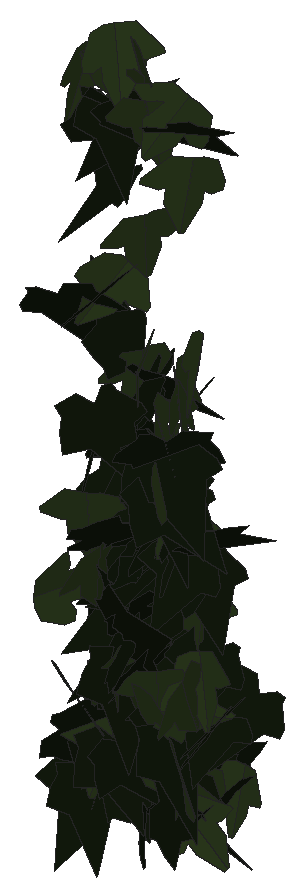
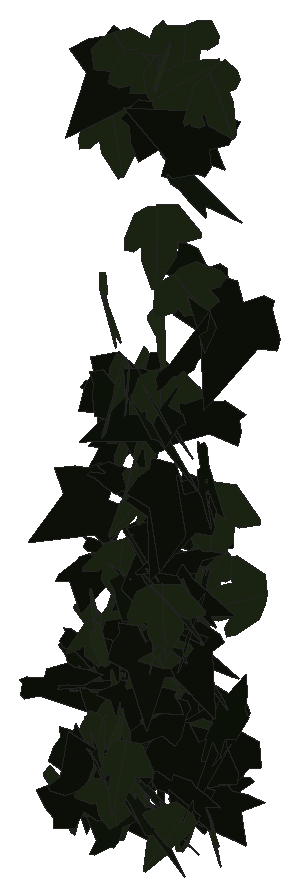
# SketchUp Ruby script. Lengths in inches.
U = 1.inch
M = Sketchup.active_model
def pt(a) = Geom::Point3d.new(a.map { |v| v * U })
def face(e, loops, mat)
  f = e.add_face(loops[0].map { |a| pt(a) })
  loops[1..].each { |l| e.add_face(l.map { |a| pt(a) }).erase! }
  f.material = f.back_material = mat if mat
  f
end
# faces: each face lists its corners as indices into pts; further lists are holes
def faces(e, pts, list, mat = nil) = list.each { |f| face(e, (f[0].is_a?(Array) ? f : [f]).map { |l| l.map { |i| pts[i] } }, mat) }
# xy, xz, yz: faces in a plane at the given z, y or x. An outline is a flat list of corners, or four numbers for a rectangle; further outlines are holes
def ring(l) = l.size == 4 ? [[l[0], l[1]], [l[2], l[1]], [l[2], l[3]], [l[0], l[3]]] : l.each_slice(2).to_a
def flat(e, list, mat, &to3) = list.each { |f| face(e, (f[0].is_a?(Array) ? f : [f]).map { |l| ring(l).map { |u, v| to3.(u, v) } }, mat) }
def xy(e, z, list, mat = nil) = flat(e, list, mat) { |x, y| [x, y, z] }
def xz(e, y, list, mat = nil) = flat(e, list, mat) { |x, z| [x, y, z] }
def yz(e, x, list, mat = nil) = flat(e, list, mat) { |y, z| [x, y, z] }
def lines(e, pts, list) = list.each { |a, b| e.add_line(pt(pts[a]), pt(pts[b])) }
# prism: a flat outline (further loops are holes) pulled along v
def prism(e, loops, v, mat = nil)
  f = face(e, loops, mat); d = Geom::Vector3d.new(v.map { |x| x * U })
  f.pushpull(f.normal.samedirection?(d) ? d.length : -d.length)
end
def box(e, o, s, mat = nil) = prism(e, [[o, [o[0] + s[0], o[1], o[2]], [o[0] + s[0], o[1] + s[1], o[2]], [o[0], o[1] + s[1], o[2]]]], [0, 0, s[2]], mat)
def at(x, y, z, deg = 0) = Geom::Transformation.translation(pt([x, y, z])) * Geom::Transformation.rotation(ORIGIN, Z_AXIS, deg.degrees)
def axes(o, x, y, z) = Geom::Transformation.new([*x, 0, *y, 0, *z, 0, *pt(o).to_a, 1])
def part(name) = M.definitions.add(name)
# library, detail: a bought-in or finely detailed component or shape, given as its bounding box
def library(name, o, s) = part(name).tap { |d| box(d.entities, o, s) }
def detail(e, o, s) = box(e.add_group.entities, o, s)
def put(e, d, t, mat = nil) = e.add_instance(d, t).tap { |i| i.material = mat if mat }
def group(e, t, mat = nil) = e.add_group.tap { |g| g.transformation = t; g.material = mat if mat }.entities
root = M.entities
M.materials.add("efeu1").color = [18, 25, 13]
M.materials.add("efeu2").color = [43, 57, 29]
c1 = part("ivyleaf_10")
p = [[0,0.5,-0.03],[-0.0625,2.02,-0.43],[-0.19,2.01,-0.46],[-0.54,1.05,-0.29],[-0.52,0.625,-0.18],[-0.83,0.76,-0.28],
  [-1.16,0.64,-0.33],[-1.15,0.33,-0.24],[-0.77,-0.39,0.02],[-0.3,-0.51,0.16],[0.04,-0.48,0.23],[-0.02,2.01,-0.4375],
  [-0.06,2.01,-0.43],[0.04,-0.49,0.23],[0.67,-0.49,0.14],[1.38,0.36,-0.2],[1.375,0.51,-0.24],[0.81,0.65,-0.19],
  [0.62,0.59,-0.15],[0.6,1.09,-0.28],[0.5,1.23,-0.31]]
faces(c1.entities,p,[[0,1,2,3,4,5,6,7,8,9,10],[11,12,0,13,14,15,16,17,18,19,20]],"efeu2")
c2 = part("ivyleaf_9")
p = [[1.54,2.16,1.25],[1.36,2.04,1.19],[-0.21,0.99,0.68],[-0.71,1.11,0.82],[-0.85,0.86,0.67],[-0.8,0.17,0.21],
  [-0.9,-0.01,0.1],[-0.67,-0.16,-0.02],[-0.08,-0.08,-0.05],[-0.03,-0.6,-0.4],[0.65,-0.88,-0.66],[0.83,-0.6,-0.49],
  [1.29,-0.42,-0.43],[1.8125,-0.07,-0.26],[1.21,0.44,0.15]]
faces(c2.entities,p,[[0,1,2,3,4,5,6,7,8,9,10,11,12,13,14]],"efeu1")
put(root,c1,axes([508.91,134.22,207.48],[0.07423,-0.16001,0.86851],[0.80996,-0.33502,-0.13095],[0.35196,0.80472,0.11818]))
put(root,c2,axes([507.8,133.62,208.01],[0.11831,-0.39809,-0.6276],[-0.20093,0.57427,-0.4291],[0.75448,0.21536,-0.01586]))
put(root,c2,axes([508.98,133.91,216.08],[-0.3317,-0.45635,-0.68755],[0.43548,0.53262,-0.56362],[0.70095,-0.54686,0.02481]))
put(root,c1,axes([509.25,134.13,225.49],[-0.6906,-0.18966,0.46272],[-0.35719,-0.36669,-0.65691],[0.38114,-0.68731,0.22278]))
put(root,c2,axes([509.09,133.77,216.5],[0.29458,0.70969,-0.45704],[-0.17433,-0.42249,-0.76839],[-0.82592,0.34229,-0.00082]))
put(root,c2,axes([508.82,134.18,208.125],[0.26109,-0.8056,-0.07748],[0.01391,0.08587,-0.84593],[0.80919,0.25846,0.03954]))
put(root,c2,axes([507.125,133.5,219.87],[0.01479,0.72128,0.2286],[-0.09256,0.21991,-0.74492],[-0.80908,-0.01198,0.08939]))
put(root,c2,axes([506.97,134.36,224.48],[0.10362,-0.76949,0.12595],[0.12525,-0.10655,-0.79964],[0.8319,0.11189,0.10471]))
put(root,c1,axes([506.6,133.95,213.91],[-0.7717,-0.40321,0.02628],[-0.02019,-0.01811,-0.87067],[0.40356,-0.77194,0.00669]))
put(root,c1,axes([508.44,133.93,225.17],[-0.80354,-0.28566,-0.0758],[0.07155,0.03079,-0.82884],[0.31025,-0.74695,-0.00518]))
put(root,c2,axes([506.76,134.02,216.58],[-0.19367,-0.35504,-0.67711],[0.46638,0.49455,-0.40418],[0.65111,-0.45985,0.0881]))
put(root,c2,axes([507.32,134.375,210.48],[0.05686,-0.19691,0.83951],[0.58416,-0.61006,-0.18266],[0.63427,0.57951,0.09297]))
put(root,c2,axes([508.81,133.95,215.19],[0.25073,-0.63994,-0.56159],[0.03991,0.59362,-0.65862],[0.85047,0.16081,0.19647]))
put(root,c2,axes([506.22,134.36,206.1],[0.02202,-0.72865,-0.08993],[-0.00532,0.08636,-0.75808],[0.79244,0.02083,-0.00259]))
put(root,c1,axes([509.48,133.875,209.94],[0.08562,-0.75709,-0.40232],[0.0693,0.40911,-0.75512],[0.85454,0.04267,0.10154]))
put(root,c1,axes([508.06,134.01,209.23],[-0.71655,0.27292,-0.01657],[0.01427,-0.00976,-0.7461],[-0.29491,-0.66359,0.00415]))
put(root,c1,axes([505.75,133.56,211.375],[0.05687,-0.0896,0.80234],[0.06874,0.77115,0.08862],[-0.83598,0.05731,0.06187]))
put(root,c2,axes([507.23,134.48,209.44],[0.0295,-0.859,-0.03641],[-0.00132,0.03639,-0.85951],[0.85977,0.02953,-0.00007]))
put(root,c2,axes([507.29,134.48,222.96],[-0.74424,0.14151,-0.32698],[0.2511,-0.32814,-0.68358],[-0.27497,-0.68268,0.26079]))
put(root,c2,axes([505.88,133.74,219.42],[0.65487,0.57749,-0.19298],[-0.15936,-0.11098,-0.87285],[-0.58766,0.67363,0.02164]))
put(root,c2,axes([509.08,133.62,206.85],[0.39514,-0.0654,-0.75758],[-0.53964,0.57738,-0.33131],[0.53572,0.62984,0.22505]))
put(root,c2,axes([506.71,133.67,213.15],[0.54201,0.07824,0.58055],[0.47797,0.40819,-0.4733],[-0.37702,0.62996,0.23458]))
put(root,c2,axes([505.71,134.62,208.07],[0.11327,-0.43365,0.71974],[0.40691,-0.60711,-0.42983],[0.73519,0.40283,0.12701]))
put(root,c1,axes([508.91,133.92,215.49],[-0.23191,0.83815,0.18605],[-0.02839,0.18512,-0.86937],[-0.85808,-0.23265,-0.02152]))
put(root,c1,axes([509.35,134.34,223.73],[-0.4995,-0.62938,0.13505],[0.03185,-0.1806,-0.80114],[0.69332,-0.44514,0.13409]))
put(root,c1,axes([507.25,134.16,226.59],[0.44874,0.67196,0.01294],[0.00647,0.01093,-0.82164],[-0.72581,0.41554,0.00068]))
put(root,c2,axes([507.6875,134.55,224.68],[-0.02293,0.31908,-0.74193],[-0.01644,-0.71369,-0.33151],[-0.84385,0.00524,0.02662]))
put(root,c1,axes([508.65,134.09,216.91],[-0.44238,0.6275,0.07194],[-0.0545,0.04965,-0.77918],[-0.67963,-0.41243,0.01566]))
put(root,c1,axes([508.39,134.29,209.63],[-0.55028,-0.50121,-0.00448],[-0.00016,0.0063,-0.74329],[0.54132,-0.5095,-0.00477]))
put(root,c1,axes([508.2,133.9,218.01],[-0.05812,0.34774,0.70288],[-0.61251,0.4327,-0.2785],[-0.54648,-0.52196,0.2374]))
put(root,c2,axes([506.32,134.75,206.13],[-0.59786,-0.59185,-0.04026],[0.02571,0.03126,-0.84125],[0.59266,-0.59839,-0.00412]))
put(root,c1,axes([506.22,134.39,225.68],[0.06928,0.74954,-0.23139],[-0.29035,-0.18848,-0.74098],[-0.79293,0.13451,0.25111]))
put(root,c1,axes([506.59,134.25,212.38],[-0.05787,-0.83776,-0.20724],[-0.00989,0.20834,-0.83943],[0.86296,-0.05379,-0.02352]))
put(root,c1,axes([507.59,134.49,225.05],[-0.53774,0.04795,-0.61741],[-0.64086,-0.10641,0.50865],[-0.05526,0.76748,0.1091]))
put(root,c2,axes([507.56,134.67,205.09],[-0.04214,0.15075,0.73136],[0.10161,-0.69714,0.16086],[0.77007,0.10023,0.0188]))
put(root,c2,axes([507.36,134.39,210.3125],[-0.73752,0.43604,-0.11187],[0.10007,-0.05055,-0.85675],[-0.4389,-0.74424,-0.00736]))
put(root,c2,axes([505.98,133.77,207.69],[0.08262,0.43541,-0.66787],[0.08949,0.63702,0.45945],[0.83315,-0.1116,0.01687]))
put(root,c1,axes([509.33,134.6,218.78],[0.54948,-0.50375,0.27163],[0.22179,-0.16355,-0.74411],[0.57129,0.54802,0.02762]))
put(root,c1,axes([506.76,134.68,207.55],[-0.49464,-0.60979,0.32314],[0.00775,-0.40246,-0.7476],[0.69008,-0.43258,0.24002]))
put(root,c2,axes([509.15,133.86,224.99],[0.7298,0.41524,0.08792],[-0.0278,0.19905,-0.80283],[-0.45681,0.65127,0.18932]))
put(root,c2,axes([506.96,134.51,207.35],[0.05756,-0.77535,-0.3381],[0.11576,0.34291,-0.76668],[0.8379,0.00589,0.12914]))
put(root,c1,axes([506.99,134.58,220.02],[0.4882,0.42536,-0.45111],[-0.4317,-0.1989,-0.63608],[-0.49409,0.59407,0.11003]))
put(root,c2,axes([510.03,134.46,208.95],[-0.47507,0.59544,-0.25634],[0.01675,-0.28856,-0.75376],[-0.69579,-0.4135,0.15687]))
put(root,c1,axes([507.67,134.49,226.24],[-0.50691,0.60483,-0.20021],[0.12507,-0.1538,-0.7962],[-0.674,-0.48342,0.00283]))
put(root,c1,axes([509.04,134.76,207.04],[-0.57058,-0.57376,0.24648],[-0.08019,-0.26378,-0.79969],[0.61929,-0.56279,0.12354]))
put(root,c2,axes([507.58,134,209.32],[0.26253,0.24345,0.66378],[0.27248,0.59756,-0.33699],[-0.68559,0.33072,0.12025]))
put(root,c2,axes([506.6,134.2,223.76],[0.01044,-0.03363,0.82332],[0.77564,0.33484,0.00567],[-0.36152,0.71742,0.03595]))
put(root,c2,axes([508.39,134.53,207.83],[0.4019,-0.46045,-0.40133],[-0.2619,0.30019,-0.61571],[0.59363,0.44417,0.00007]))
put(root,c1,axes([507.3125,134.27,209.4],[-0.17461,0.52695,0.48182],[-0.33829,0.37122,-0.5528],[-0.67808,-0.32089,0.15172]))
put(root,c1,axes([509.19,134.45,206.14],[0.46271,0.36201,0.46722],[0.35744,0.30414,-0.58313],[-0.51039,0.54119,0.01519]))
put(root,c1,axes([506.1,134.86,206.12],[0.57016,-0.61617,0.07402],[0.04947,-0.05507,-0.83949],[0.61863,0.5723,-0.00108]))
put(root,c2,axes([506.08,134.98,215.4],[-0.40571,0.18413,-0.63651],[0.59063,-0.2748,-0.43508],[-0.35723,-0.66346,0.00356]))
put(root,c1,axes([507.67,134.7,221.52],[-0.39786,-0.66242,-0.08049],[0.04787,0.0639,-0.78825],[0.71869,-0.37097,0.00795]))
put(root,c2,axes([508.24,134.67,208.48],[0.43003,-0.66202,-0.32096],[-0.00404,0.36964,-0.76783],[0.73571,0.38898,0.18339]))
put(root,c2,axes([509.55,134.74,208.38],[-0.44636,0.54078,-0.16379],[0.04251,-0.16712,-0.70427],[-0.60682,-0.4095,0.07113]))
put(root,c1,axes([509.15,134.88,209.99],[0.71102,-0.03826,0.27967],[0.29112,0.00523,-0.68555],[0.03611,0.71114,0.02009]))
put(root,c1,axes([508.08,135.08,208.4],[0.27302,0.49705,-0.41391],[-0.20376,-0.35051,-0.57989],[-0.65682,0.31535,0.00785]))
put(root,c1,axes([508.76,134.45,208.9],[-0.09113,-0.22723,-0.71314],[0.53431,0.48487,-0.23042],[0.56848,-0.49215,0.10225]))
put(root,c1,axes([507.11,134.5,209.6],[-0.26232,-0.5787,-0.57867],[0.24051,0.52633,-0.63537],[0.78225,-0.35588,0.0013]))
put(root,c2,axes([508.2,134.37,207.95],[0.20866,0.60973,0.32272],[0.10251,0.29544,-0.6652],[-0.73174,0.21526,-0.00116]))
put(root,c2,axes([508.12,134.66,207.39],[0.48794,0.49387,-0.21188],[-0.13892,-0.1584,-0.69602],[-0.56,0.46961,-0.01195]))
put(root,c2,axes([507.61,135.12,217.15],[-0.67517,0.24099,-0.32427],[0.30845,-0.1258,-0.69666],[-0.29325,-0.68718,0.01381]))
put(root,c2,axes([506.875,134.95,217.81],[-0.27565,-0.63084,0.36355],[0.1396,0.3248,0.70773],[-0.76631,0.28609,-0.00184]))
put(root,c2,axes([508.59,135.35,212.59],[-0.65488,-0.34195,-0.13833],[0.1881,-0.04212,-0.71314],[0.34877,-0.61936,0.12487]))
put(root,c2,axes([506.99,135.3,210.67],[-0.71938,-0.11925,0.19816],[-0.20094,-0.04189,-0.7037],[0.13622,-0.69154,0.00845]))
put(root,c2,axes([508.58,135.01,205.95],[0.64863,-0.26276,0.26668],[0.25466,-0.10078,-0.68177],[0.30393,0.64521,0.00212]))
put(root,c2,axes([507.76,135.32,213.89],[0.26629,-0.69149,0.05696],[0.03335,-0.04713,-0.76337],[0.7484,0.24814,0.01375]))
put(root,c2,axes([508.5625,135.38,214.56],[-0.74695,-0.08633,0.25258],[-0.24679,-0.11637,-0.71979],[0.12878,-0.72372,0.0856]))
put(root,c2,axes([509.21,135.52,208.61],[-0.42095,-0.5809,-0.02417],[0.20602,-0.10136,-0.6924],[0.59312,-0.37707,0.22335]))
put(root,c2,axes([506.13,134.89,206.31],[-0.14162,-0.54631,0.62467],[0.15468,0.60522,0.56436],[-0.81531,0.20971,-0.00144]))
put(root,c1,axes([508.47,135.04,217.15],[-0.59029,0.52685,-0.01494],[-0.07362,-0.09119,-0.78073],[-0.56443,-0.5391,0.11746]))
put(root,c2,axes([508.44,134.53,206.42],[0.31142,0.44284,0.47144],[0.20168,0.41654,-0.54673],[-0.65403,0.33931,0.05589]))
put(root,c2,axes([506.44,134.71,207.54],[0.27075,0.80063,-0.08179],[-0.01382,-0.08166,-0.84507],[-0.80468,0.27079,-0.01301]))
put(root,c2,axes([507.4375,135.5,214.51],[-0.69005,-0.31496,0.16957],[-0.14978,-0.08732,-0.74064],[0.35253,-0.65361,0.01724]))
put(root,c2,axes([507.3,134.67,210.98],[0.36491,0.58236,0.2256],[0.12037,0.18613,-0.70021],[-0.66029,0.35578,-0.00297]))
put(root,c2,axes([508.69,135.01,216.75],[-0.33091,0.68915,-0.04478],[0.01408,-0.04132,-0.78434],[-0.7456,-0.30663,0.00506]))
put(root,c1,axes([507.15,135.24,217.46],[-0.35868,-0.67113,-0.05054],[0.05095,0.03083,-0.77819],[0.72493,-0.33423,0.02969]))
put(root,c2,axes([506.11,134.91,212.22],[0.40943,-0.1091,-0.63777],[-0.59387,0.27857,-0.40508],[0.31597,0.66496,0.06506]))
put(root,c2,axes([507.09,135.04,208.78],[0.7502,0.13153,0.04406],[0.04508,0.00726,-0.73526],[-0.14226,0.69589,-0.00066]))
put(root,c2,axes([506.53,135.08,212.07],[-0.2295,0.281,0.68532],[-0.50504,0.46628,-0.36362],[-0.5861,-0.51182,0.04498]))
put(root,c2,axes([509.19,134.85,213.42],[0.5849,0.32563,0.37974],[0.21358,0.35251,-0.632],[-0.48329,0.54988,0.18027]))
put(root,c2,axes([508.65,135.52,212.1],[-0.71693,0.19831,0.14503],[-0.16422,-0.02395,-0.71733],[-0.20393,-0.67789,0.06777]))
put(root,c2,axes([509.6,135.05,206.44],[-0.03242,0.67702,0.11213],[-0.02307,0.10694,-0.70459],[-0.74004,-0.03299,0.01705]))
put(root,c2,axes([506.9375,134.94,212.83],[0.47773,0.48491,0.30214],[0.22863,0.19995,-0.6823],[-0.56607,0.48999,-0.02059]))
put(root,c2,axes([507.81,135.55,213.26],[-0.66593,0.32001,-0.18091],[0.17234,-0.07012,-0.72239],[-0.35361,-0.63682,-0.01137]))
put(root,c2,axes([506.43,135.4375,210.95],[-0.02632,0.59359,-0.40428],[-0.10505,-0.38808,-0.60997],[-0.75908,0.03313,0.09843]))
put(root,c2,axes([507.47,135.46,216.79],[-0.62604,0.4564,-0.03242],[0.01735,-0.02999,-0.76716],[-0.49376,-0.57973,0.01415]))
put(root,c1,axes([508.37,135.11,217.21],[0.19345,-0.48483,-0.57878],[0.05505,0.57943,-0.50792],[0.79523,0.07783,0.17596]))
put(root,c2,axes([508.96,135.74,210.01],[-0.66103,-0.26463,-0.25416],[0.2422,0.09711,-0.6935],[0.30444,-0.65186,-0.00014]))
put(root,c1,axes([507.71,135.11,215.6],[0.13005,-0.44766,-0.60911],[0.03772,0.59624,-0.4665],[0.79525,0.04493,0.12173]))
put(root,c2,axes([507.63,135.89,211.17],[-0.11442,-0.18013,-0.70496],[-0.34361,-0.5986,0.21715],[-0.67506,0.33522,0.00896]))
put(root,c2,axes([507.04,135.25,216.93],[0.75041,0.01458,0.25124],[0.2561,0.10584,-0.71595],[-0.05226,0.72797,0.09906]))
put(root,c2,axes([508.64,135.7,212.33],[-0.0987,-0.64688,-0.33854],[0.05305,0.3218,-0.67943],[0.78029,-0.10371,0.00337]))
put(root,c2,axes([506.2,136.03,213.34],[-0.37305,-0.62294,0.013],[0.12835,-0.0799,-0.72578],[0.66056,-0.33628,0.14836]))
put(root,c2,axes([507.89,135.34,206.58],[-0.12828,0.46472,0.49369],[-0.39338,0.35772,-0.45899],[-0.59999,-0.33389,0.19538]))
put(root,c2,axes([507.03,135.4,211.98],[-0.30907,0.50876,0.42059],[-0.36038,0.26418,-0.5912],[-0.60233,-0.41912,0.1379]))
put(root,c2,axes([507.46,135.58,206.14],[-0.47958,0.37839,0.372],[-0.33219,0.18869,-0.60472],[-0.45375,-0.53807,0.04954]))
put(root,c2,axes([506.12,135.99,207.22],[-0.67608,-0.17169,-0.18229],[0.18793,0.02795,-0.67481],[0.18682,-0.64947,0.01915]))
put(root,c2,axes([506.39,135.41,215.07],[0.34438,0.63359,-0.0514],[-0.02716,-0.04267,-0.73767],[-0.68581,0.31984,0.00341]))
put(root,c2,axes([508.46,135.55,207.5],[-0.33568,0.57839,0.17505],[-0.17864,0.10018,-0.67566],[-0.62557,-0.33897,0.09901]))
put(root,c2,axes([509.84,136.21,208.89],[-0.52562,-0.50018,0.05346],[-0.05074,-0.02598,-0.72562],[0.54066,-0.4887,-0.01613]))
put(root,c2,axes([507.43,135.77,212.07],[-0.37167,0.60411,-0.14566],[-0.08639,-0.20208,-0.7021],[-0.66415,-0.31178,0.17284]))
put(root,c1,axes([507.92,135.78,212.95],[0.23314,0.68063,-0.00646],[-0.0214,-0.00023,-0.74235],[-0.7348,0.21596,0.01957]))
put(root,c1,axes([507.7,136.1,208.7],[0.36479,-0.21279,0.60894],[0.58647,-0.22588,-0.41116],[0.32977,0.6371,0.0576]))
put(root,c2,axes([506.25,135.53,214.83],[0.54864,0.48507,-0.10739],[-0.07326,-0.07846,-0.73042],[-0.53058,0.51241,-0.01018]))
put(root,c2,axes([507.77,136.21,206.14],[-0.63675,-0.35583,-0.01666],[0.01538,0.00741,-0.71618],[0.38438,-0.58975,0.00106]))
put(root,c1,axes([507.34,135.48,214.65],[-0.00873,0.32678,0.67742],[-0.10003,0.64566,-0.33807],[-0.78065,-0.08639,0.03574]))
put(root,c1,axes([506.88,136.03,210.92],[-0.51214,0.45112,-0.21636],[0.16743,-0.13886,-0.68066],[-0.50973,-0.49887,-0.00619]))
put(root,c1,axes([506.44,136.08,212.18],[-0.57781,-0.45308,0.05174],[-0.01593,-0.05946,-0.72818],[0.49201,-0.53401,0.03718]))
put(root,c1,axes([506.42,136.26,210.66],[0.36989,0.50352,-0.35744],[-0.20361,-0.28742,-0.6333],[-0.62614,0.39092,-0.00522]))
put(root,c2,axes([506.99,136.2,209.52],[-0.26944,-0.47998,-0.42645],[0.28385,0.3219,-0.55818],[0.61988,-0.35603,0.07023]))
put(root,c1,axes([508.32,136.15,210.91],[0.10985,0.67382,-0.15124],[-0.02306,-0.14384,-0.70872],[-0.74413,0.10393,-0.00037]))
put(root,c1,axes([508.07,136.3,210.36],[0.35764,-0.57348,-0.22869],[0.1237,-0.18777,0.68869],[-0.65169,-0.35036,0.00522]))
put(root,c1,axes([507.76,136.22,208.52],[-0.53797,0.47614,-0.1273],[0.10486,-0.07555,-0.71653],[-0.52049,-0.50734,-0.01277]))
put(root,c1,axes([509.13,136.47,206.29],[0.70588,-0.1975,0.08251],[0.08018,-0.02857,-0.71007],[0.21543,0.65777,-0.00607]))
put(root,c2,axes([507.79,136.34,207.41],[-0.49949,0.48705,-0.10097],[0.02304,-0.11306,-0.69556],[-0.53587,-0.45885,0.06421]))
put(root,c2,axes([507.17,136.73,205.99],[0.27,-0.51937,0.34146],[0.29773,-0.22198,-0.58349],[0.59306,0.34789,0.13746]))
put(root,c2,axes([507.96,136.36,207.28],[-0.49013,0.50768,0.13565],[-0.11336,0.08101,-0.70775],[-0.55463,-0.46519,0.02479]))
put(root,c1,axes([505.91,136.125,206.29],[0.17143,0.4391,0.50145],[-0.00442,0.4969,-0.46922],[-0.7043,0.10376,0.125]))
put(root,c1,axes([508.11,136.5,208.2],[-0.58519,0.42061,0.04332],[-0.07214,-0.01834,-0.71105],[-0.45074,-0.54313,0.05756]))
put(root,c2,axes([506.66,136.65,206.74],[-0.55398,0.40878,-0.09398],[0.06612,-0.06814,-0.68197],[-0.44728,-0.51637,0.01559]))
put(root,c2,axes([506.73,136.33,210.93],[-0.01368,0.69133,0.04307],[0.00426,0.04149,-0.71909],[-0.74797,-0.01241,-0.00488]))
put(root,c2,axes([508.26,136.82,206.15],[0.47233,0.37265,0.35873],[-0.30968,-0.19447,0.5966],[0.45261,-0.52195,0.03383]))
put(root,c1,axes([507.39,136.74,206.91],[0.65567,0.2912,-0.03593],[-0.06263,0.04137,-0.69725],[-0.31045,0.60667,0.06479]))
put(root,c1,axes([507.07,136.71,207.96],[-0.16266,-0.59419,-0.29436],[0.06711,0.27623,-0.63746],[0.70764,-0.16278,-0.00721]))
put(root,c2,axes([508.3,136.66,206.83],[-0.37617,-0.27409,0.53015],[0.43229,0.31565,0.46094],[-0.45149,0.5306,-0.00036]))
